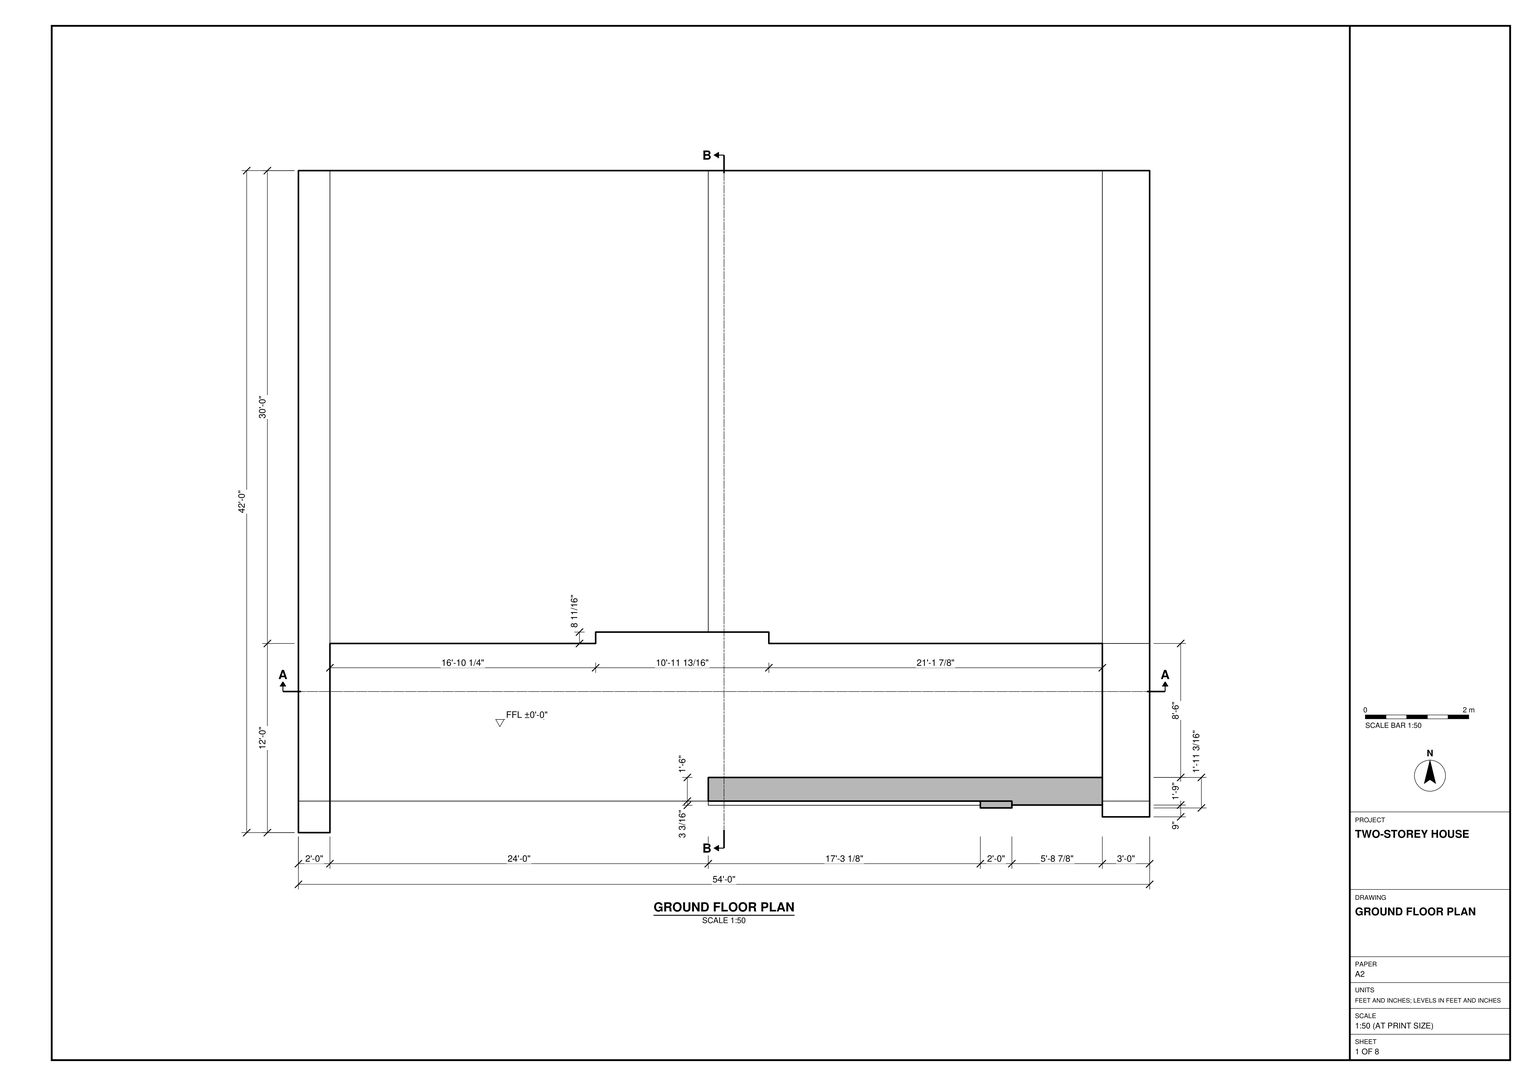
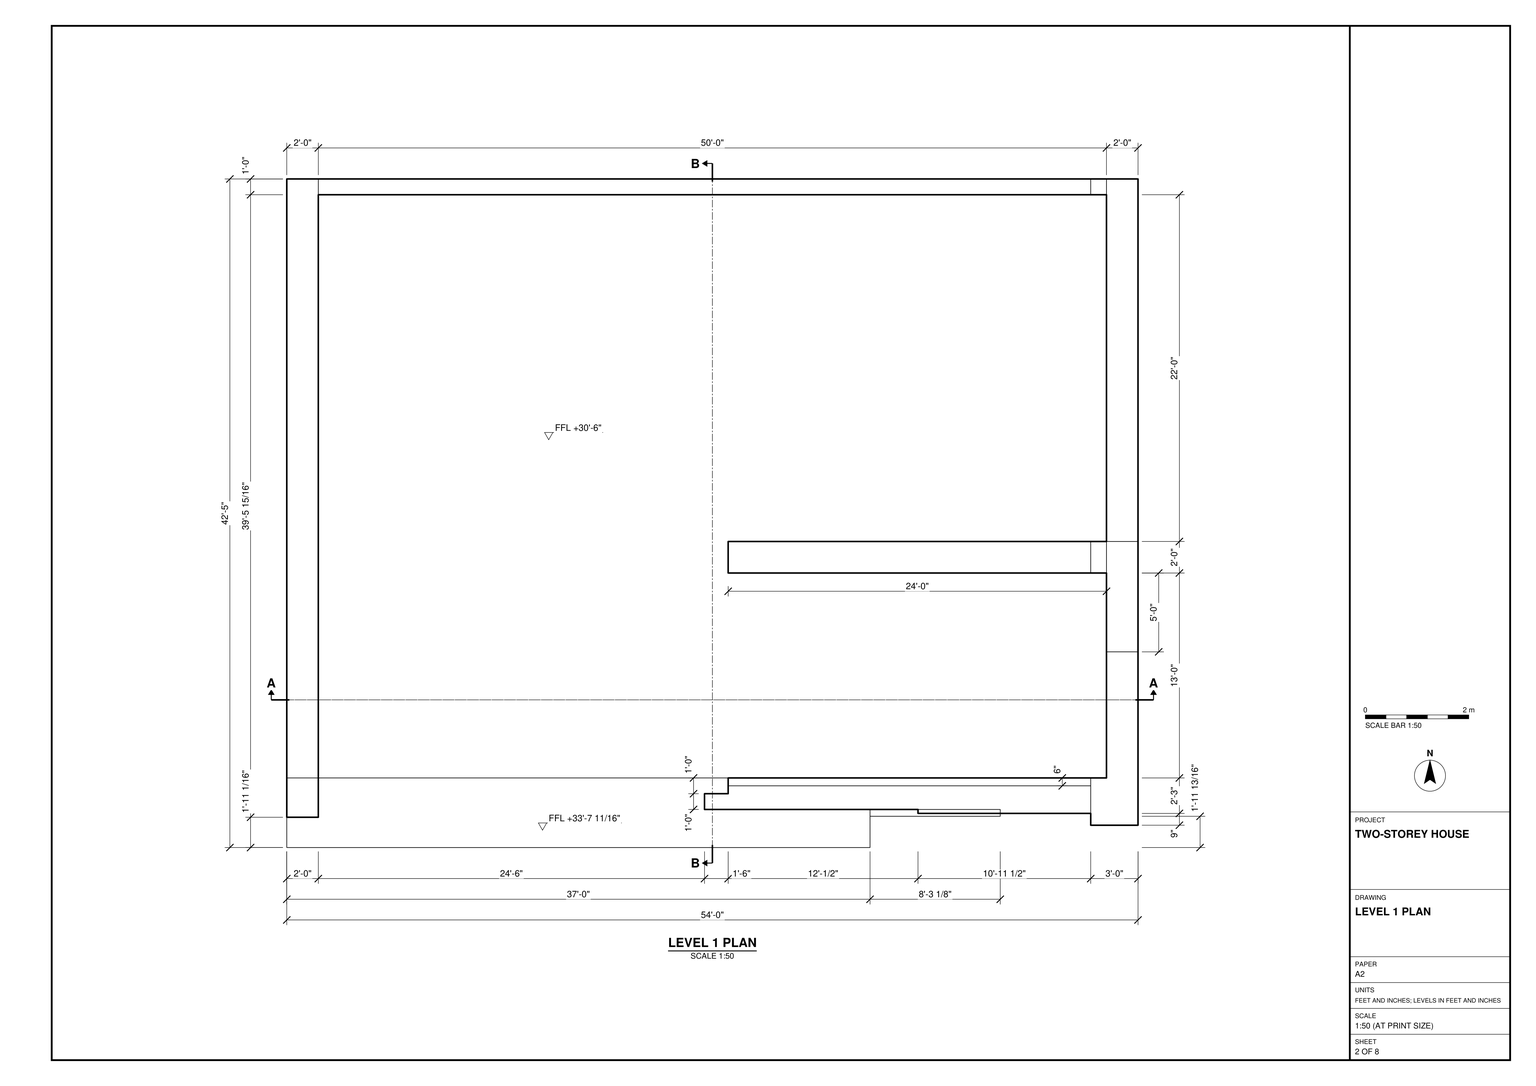
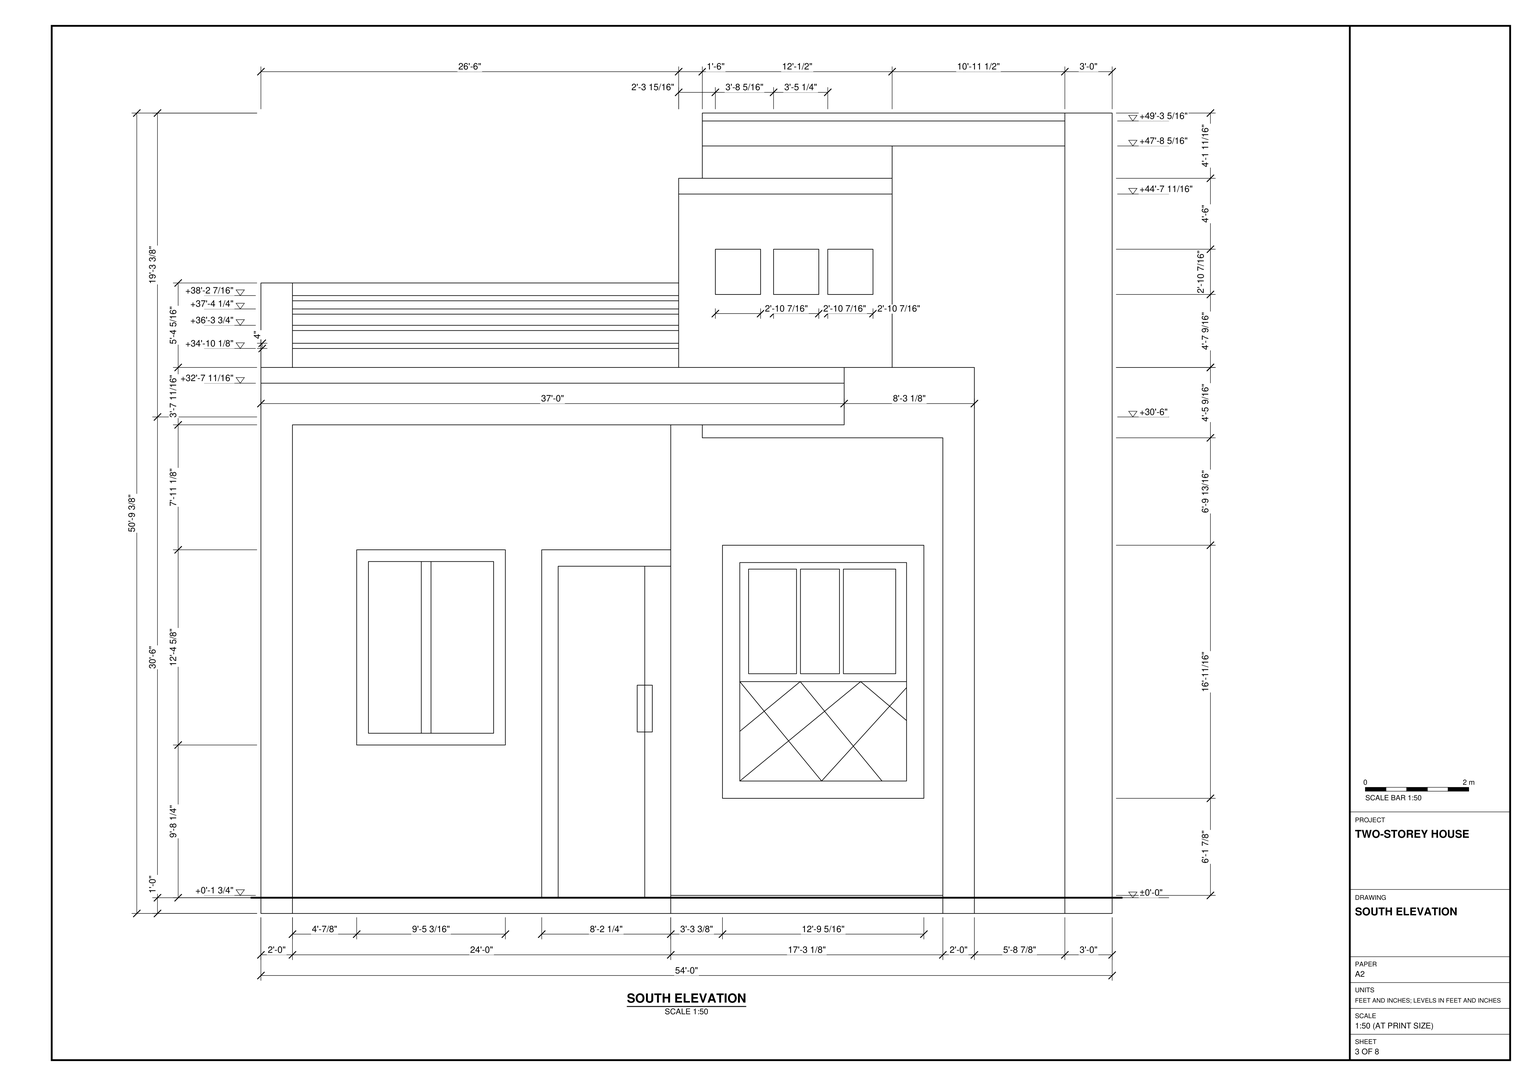
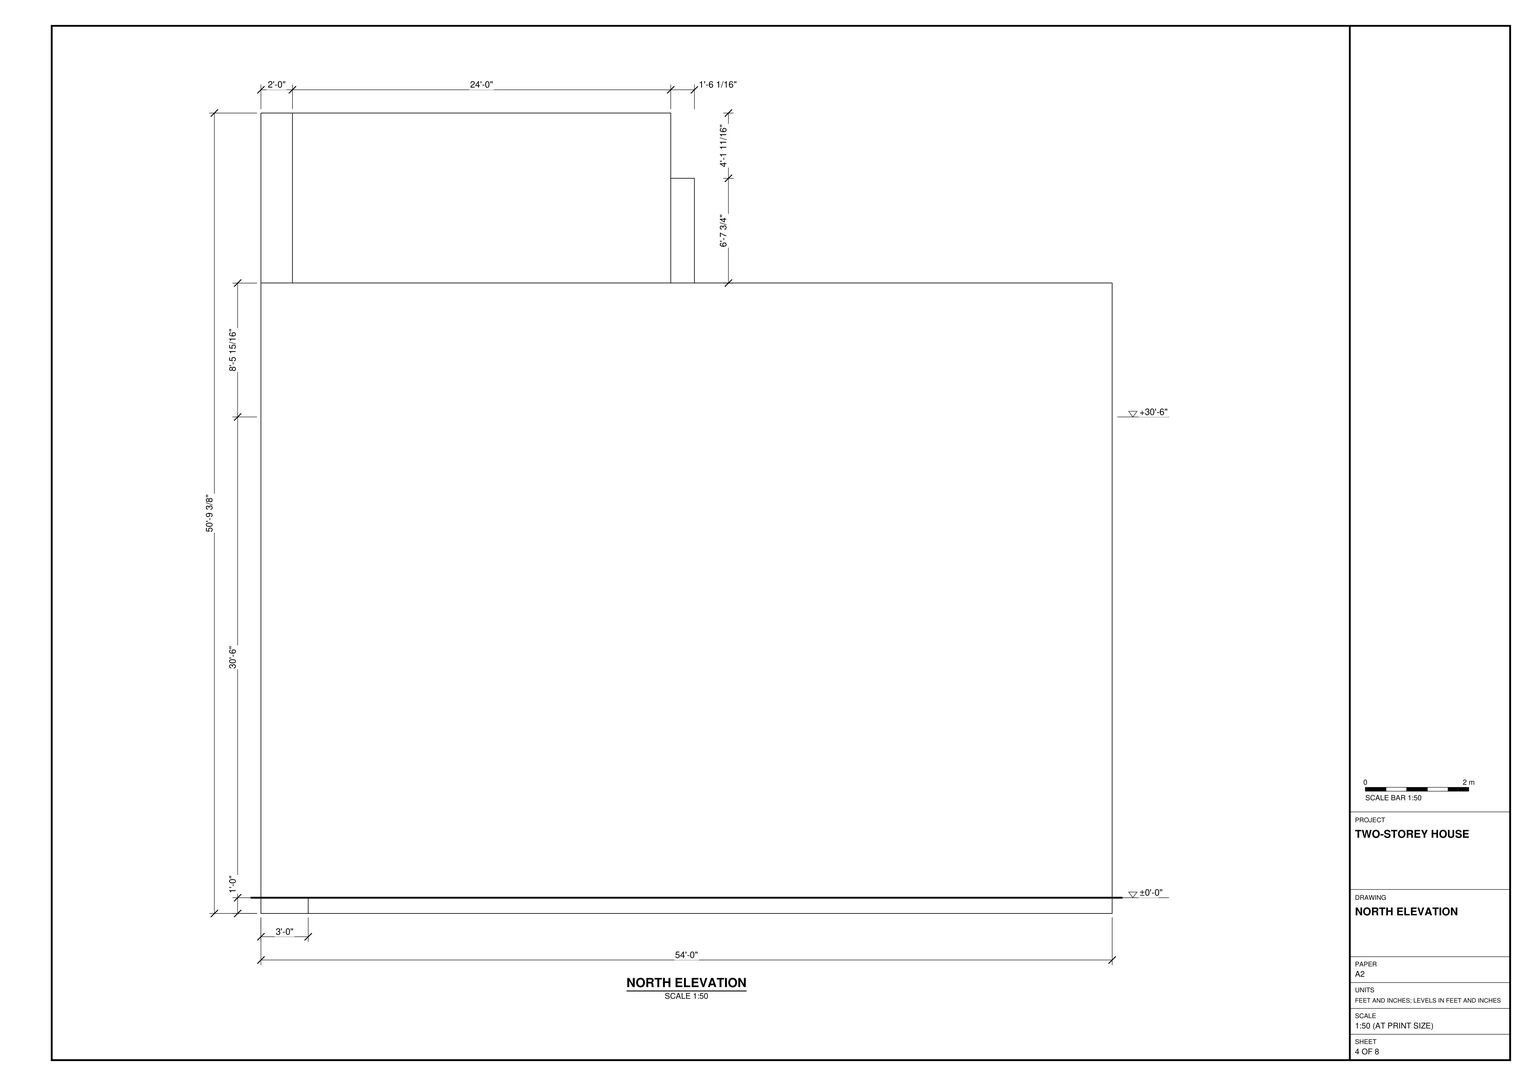
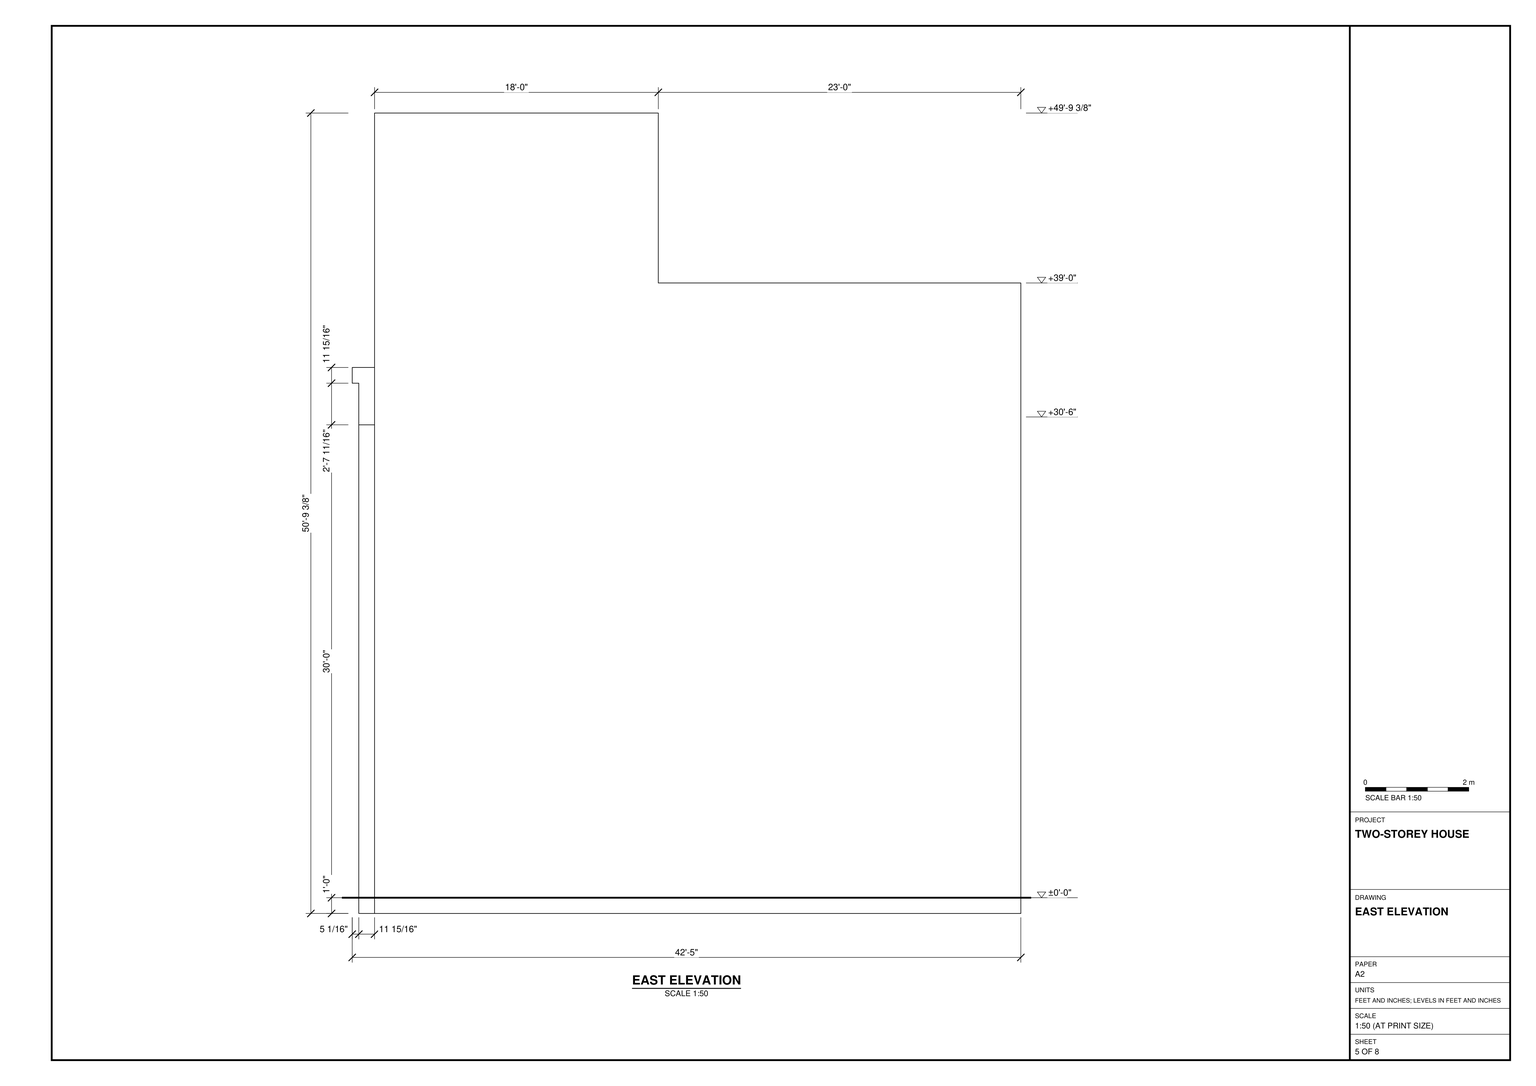
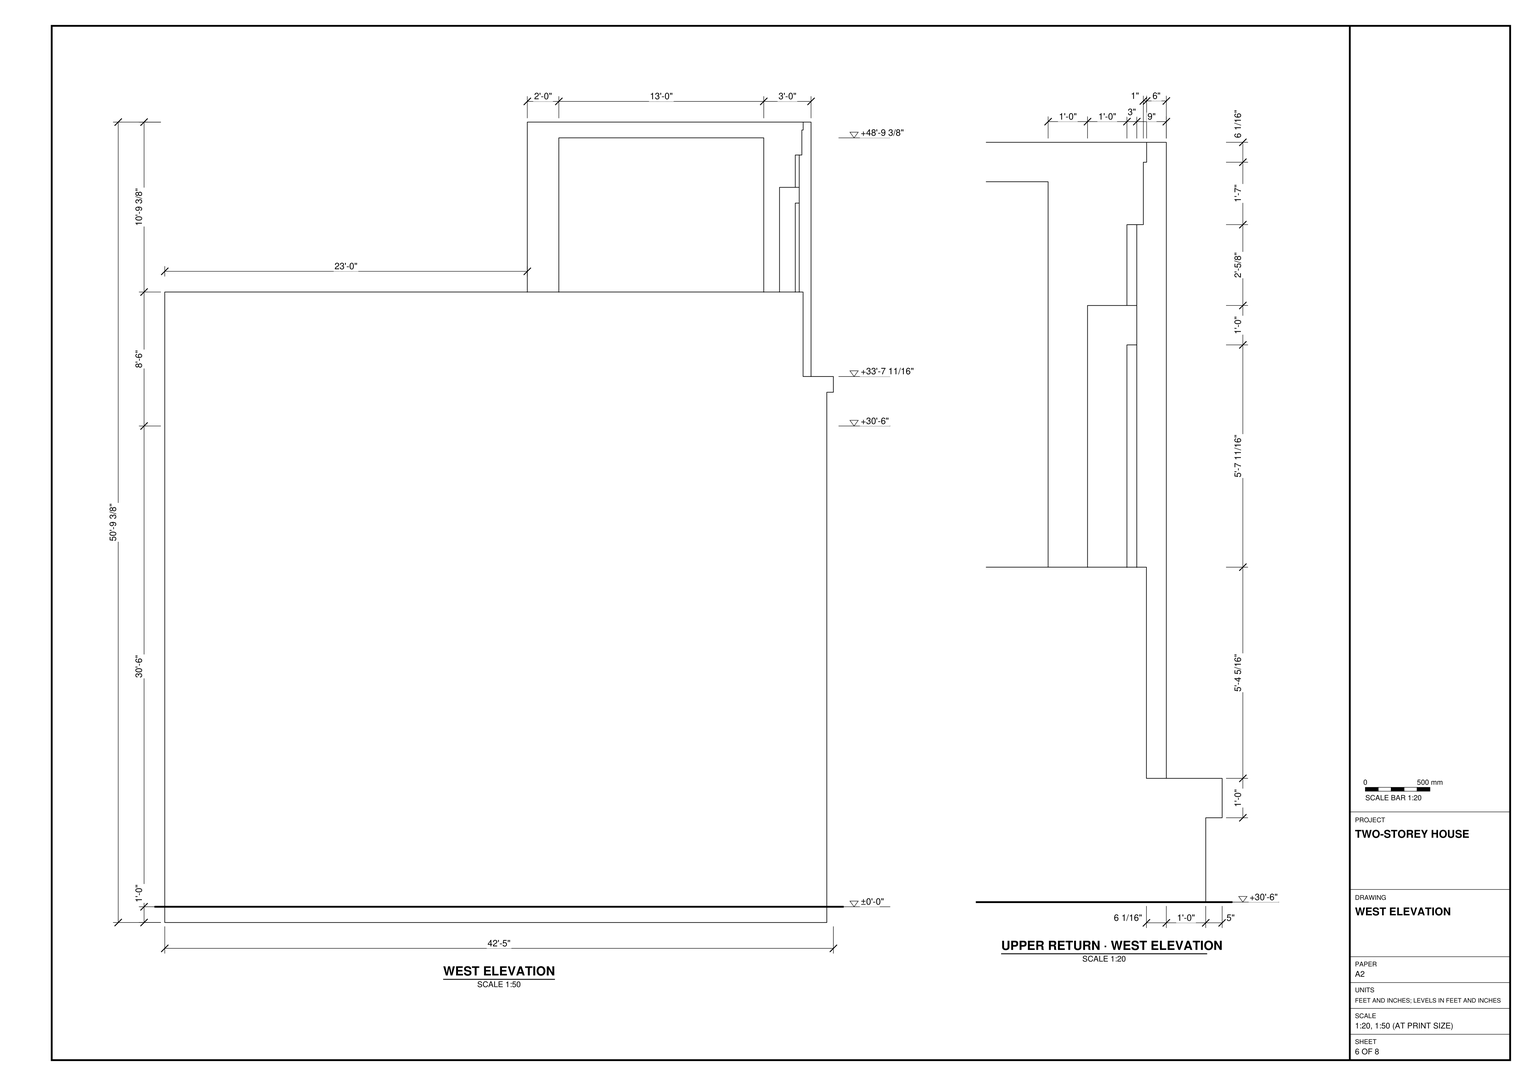
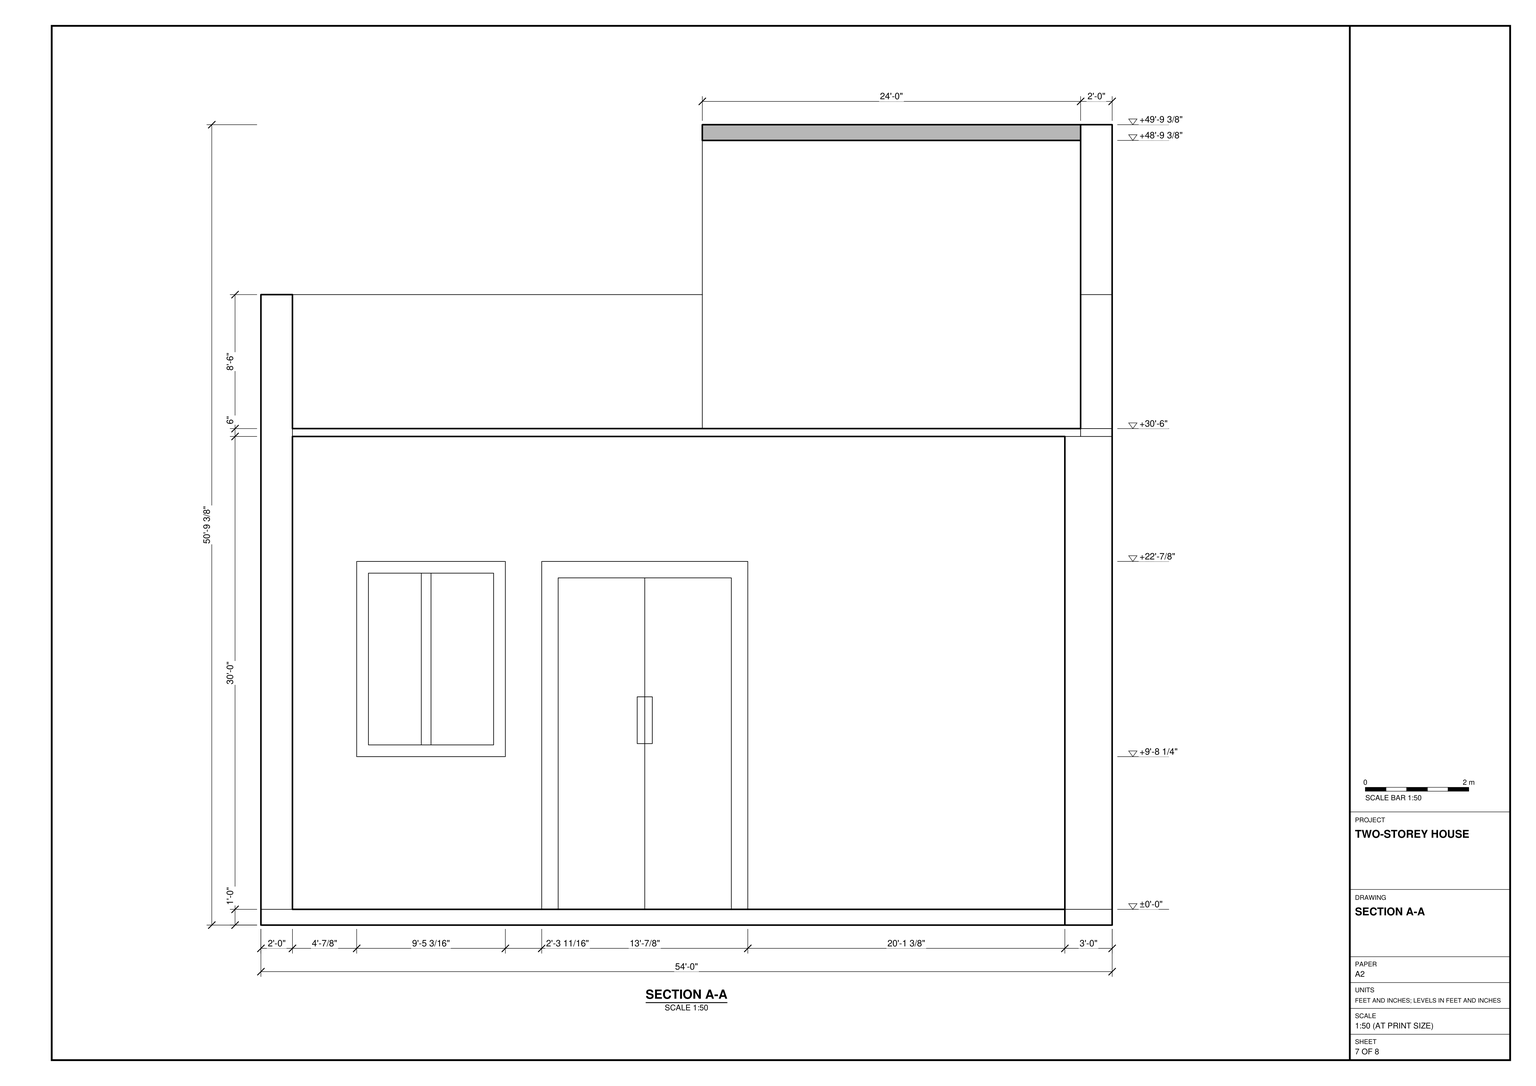
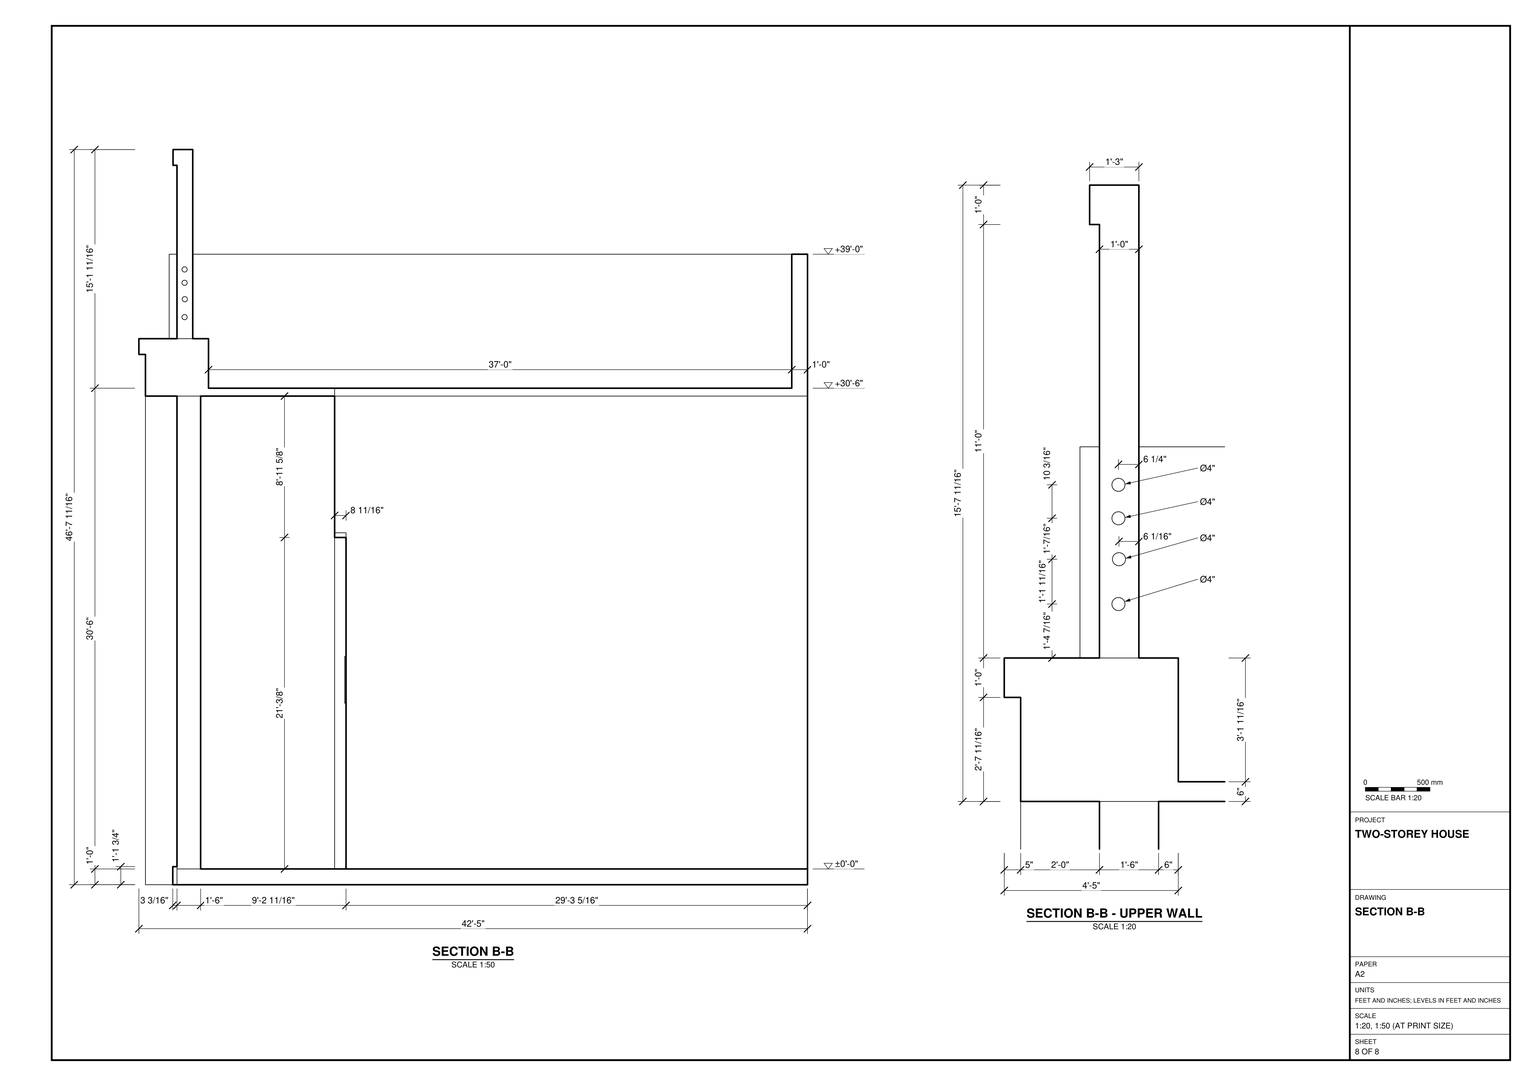
Model the house in SketchUp using task_files/diagram_01.pdf. Work in feet and inches. The overall dimensions are 54'-0" wide along X, 42'-5" deep along Y and 50'-9 3/8" high. Set the ground floor at ±0'-0" and the upper floor at +30'-6".

Use the plans to lay out the base, floor slabs and walls, following the wall thicknesses and changes in outline as drawn. On the south side, set the entrance wall back behind the side piers. Place the entrance door between the narrower divided window on the left and the larger framed window on the right. Model the upper panes and diagonal lower grille of the right-hand window. Carry the horizontal beam across the front and turn it down beside this window.

Follow the upper plan for the slab edges and the narrow return on the right. Match the stepped roof profile in the south elevation: the horizontal rails on the left meet a raised panel with three square openings, and the highest roof edge rises behind the panel to the right. Include stairs, built-in joinery and main furniture where shown. Keep shell elements such as walls, slabs and roof separate as groups or components, group each furniture or joinery piece separately, and use components for repeated parts. Decor and loose items may be any suitable library components. Save one SketchUp model as output_files/two_storey_house_with_a_stepped_south_facade.skp.

# SketchUp Ruby script. Lengths in inches.
U = 1.inch
M = Sketchup.active_model
def pt(a) = Geom::Point3d.new(a.map { |v| v * U })
def face(e, loops, mat)
  f = e.add_face(loops[0].map { |a| pt(a) })
  loops[1..].each { |l| e.add_face(l.map { |a| pt(a) }).erase! }
  f.material = f.back_material = mat if mat
  f
end
# faces: each face lists its corners as indices into pts; further lists are holes
def faces(e, pts, list, mat = nil) = list.each { |f| face(e, (f[0].is_a?(Array) ? f : [f]).map { |l| l.map { |i| pts[i] } }, mat) }
# xy, xz, yz: faces in a plane at the given z, y or x. An outline is a flat list of corners, or four numbers for a rectangle; further outlines are holes
def ring(l) = l.size == 4 ? [[l[0], l[1]], [l[2], l[1]], [l[2], l[3]], [l[0], l[3]]] : l.each_slice(2).to_a
def flat(e, list, mat, &to3) = list.each { |f| face(e, (f[0].is_a?(Array) ? f : [f]).map { |l| ring(l).map { |u, v| to3.(u, v) } }, mat) }
def xy(e, z, list, mat = nil) = flat(e, list, mat) { |x, y| [x, y, z] }
def xz(e, y, list, mat = nil) = flat(e, list, mat) { |x, z| [x, y, z] }
def yz(e, x, list, mat = nil) = flat(e, list, mat) { |y, z| [x, y, z] }
def lines(e, pts, list) = list.each { |a, b| e.add_line(pt(pts[a]), pt(pts[b])) }
# prism: a flat outline (further loops are holes) pulled along v
def prism(e, loops, v, mat = nil)
  f = face(e, loops, mat); d = Geom::Vector3d.new(v.map { |x| x * U })
  f.pushpull(f.normal.samedirection?(d) ? d.length : -d.length)
end
def box(e, o, s, mat = nil) = prism(e, [[o, [o[0] + s[0], o[1], o[2]], [o[0] + s[0], o[1] + s[1], o[2]], [o[0], o[1] + s[1], o[2]]]], [0, 0, s[2]], mat)
def at(x, y, z, deg = 0) = Geom::Transformation.translation(pt([x, y, z])) * Geom::Transformation.rotation(ORIGIN, Z_AXIS, deg.degrees)
def axes(o, x, y, z) = Geom::Transformation.new([*x, 0, *y, 0, *z, 0, *pt(o).to_a, 1])
def part(name) = M.definitions.add(name)
# library, detail: a bought-in or finely detailed component or shape, given as its bounding box
def library(name, o, s) = part(name).tap { |d| box(d.entities, o, s) }
def detail(e, o, s) = box(e.add_group.entities, o, s)
def put(e, d, t, mat = nil) = e.add_instance(d, t).tap { |i| i.material = mat if mat }
def group(e, t, mat = nil) = e.add_group.tap { |g| g.transformation = t; g.material = mat if mat }.entities
root = M.entities
M.materials.add("[0001_PaleVioletRed]").color = [219, 112, 147]
M.materials.add("[0009_Linen]").color = [186, 178, 171]
M.materials.add("[0023_FireBrick]").color = [71, 13, 13]
M.materials.add("[0035_Tan]").color = [114, 98, 76]
M.materials.add("[0042_Sienna]").color = [58, 30, 16]
M.materials.add("[0119_RosyBrown]").color = [124, 95, 95]
M.materials.add("[0134_DimGray]").color = [105, 105, 105]
M.materials.add("[0137_Black]").color = [0, 0, 0]
M.materials.add("[Asphalt New]").color = [67, 60, 62]
M.materials.add("[Granite Brown]").color = [126, 104, 91]
M.materials.add("[Translucent Glass Gray]").color = [128, 128, 128]
M.materials["[Translucent Glass Gray]"].alpha = 0.5
xy(root,0,[[0,5,24,29],[612,17,648,29],[519.125,23.8,543.125,29],[312,25.8,312,29,0,29,0,509,612,509,612,26,543.125,26,543.125,29,519.125,29,519.125,25.8],[612,29,648,509]])
xy(root,12,[[24,149,24,509,312,509,312,157.6875,226.28,157.6875,226.28,149],[358.11,149,358.11,157.6875,312,157.6875,312,509,612,509,612,149]])
xy(root,12,[[24,29,312,29,312,47,612,47,612,149,358.11,149,358.11,157.6875,226.28,157.6875,226.28,149,24,149]],"[Granite Brown]")
xy(root,13.76,[[312,25.8,519.125,29]])
xy(root,87.65,[[351.36,17,504.67,29]])
xy(root,100.83,[[364.54,17,491.5,29]])
xy(root,137.19,[[81.83,149,122.08,157.6875],[129.48,149,177.13,157.6875]])
xy(root,138.18,[[286.45,156.6875,292.2,157.6875],[292.2,156.6875,297.95,157.6875]])
xy(root,173.8,[[286.45,156.6875,292.2,157.6875],[292.2,156.6875,297.95,157.6875]])
xy(root,264.36,[[226.28,149,358.11,157.6875]])
xy(root,267.16,[[364.54,17,491.5,29]])
xy(root,267.93,[[81.83,149,122.08,157.6875],[129.48,149,177.13,157.6875]])
xy(root,280.34,[[351.36,17,504.67,29]])
xy(root,362.125,[[336,23.8,519.125,29]])
xy(root,372,[[24,5,24,149,612,149,612,47,312,47,312,29,336,29,336,23.8,444,23.8,444,5],[336,23.8,444,29]])
xy(root,378,[[24,53,624,53,624,209,336,209,336,233,624,233,624,497,24,497]])
xy(root,403.6875,[[0,0,444,5]])
xy(root,415.6875,[[444,23.8,543.125,23.8,543.125,26,480.51,26,480.51,29,444,29],[480.51,26,543.125,29]])
xy(root,415.6875,[[0,0,444,0,444,29,318,29,318,41,336,41,336,53,24,53,24,23.0625,0,23.0625]],"[Asphalt New]")
xy(root,430.13,[[24,34.5,318,35.02]])
xy(root,443.79,[[24,34.66,318,35.18]])
xy(root,460.22,[[24,34.54,318,35.06]])
xy(root,470.41,[[24,34.54,318,35.06]])
xy(root,471.25,[[345.95,29,380.38,31],[390.26,29,424.7,31],[431.51,29,465.95,31]],"[0137_Black]")
xy(root,480,[[0,23.0625,24,509],[624,233,648,233,648,509,24,509,24,497,624,497]])
xy(root,505.68,[[345.95,29,380.38,31],[390.26,29,424.7,31],[431.51,29,465.95,31]],"[0137_Black]")
xy(root,547.6875,[[318,26,480.51,29]])
xy(root,559.6875,[[318,26,480.51,26,480.51,29,336,29,336,41,318,41]])
xy(root,584.3125,[[336,24,336,29,480.51,29,480.51,26,612,26,612,24],[480.51,26,612,29]])
xy(root,597.375,[[336,53,624,209]])
xy(root,603.3125,[[336,23,612,24]])
xy(root,609.375,[[612,17,648,17,648,233,336,233,336,209,624,209,624,53,336,53,336,23,612,23],[336,53,624,209]])
xz(root,0,[[0,403.6875,444,415.6875]],"[Asphalt New]")
xz(root,5,[[0,0,24,0,24,372,444,372,444,403.6875,0,403.6875]],"[Asphalt New]")
xz(root,17,[[[351.36,87.65,504.67,280.34],[364.54,100.83,491.5,267.16]]],"[0035_Tan]")
xz(root,17,[[612,0,648,609.375]],"[Asphalt New]")
xz(root,23,[[336,603.3125,612,609.375]],"[Asphalt New]")
xz(root,23.0625,[[0,415.6875,24,480]])
xz(root,23.8,[[519.125,0,543.125,0,543.125,415.6875,444,415.6875,444,372,336,372,336,362.125,519.125,362.125]],"[0001_PaleVioletRed]")
xz(root,24,[[336,584.3125,612,603.3125]],"[Asphalt New]")
xz(root,25.8,[[312,0,519.125,13.76]],"[0134_DimGray]")
xz(root,26,[[318,547.6875,480.51,559.6875]])
xz(root,26,[[543.125,0,612,0,612,584.3125,480.51,584.3125,480.51,415.6875,543.125,415.6875]],"[0119_RosyBrown]")
xz(root,29,[[519.125,0,519.125,362.125,336,362.125,336,372,444,372,444,415.6875,543.125,415.6875,543.125,0],[[351.36,87.65,504.67,280.34],[364.54,100.83,491.5,267.16]],[371.23,182.52,407.73,262.16],[410.73,182.52,440.42,262.16],[443.42,182.52,483.25,262.16]])
xz(root,29,[[[312,13.76,519.125,13.76,519.125,362.125,336,362.125,336,372,312,372],[351.36,87.65,504.67,280.34]],[[318,415.6875,480.51,547.6875],[345.95,471.25,380.38,505.68],[390.26,471.25,424.7,505.68],[431.51,471.25,465.95,505.68]],[336,559.6875,480.51,584.3125]],"[0001_PaleVioletRed]")
xz(root,29,[[364.54,100.83,401.68,131.38,383.11,153.95,365.93,139.8125,364.54,138.67],[364.54,100.83,426.82,100.83,401.68,131.38],[426.82,100.83,450.96,127.39,429.1,153.95,401.68,131.38],[426.82,100.83,472.8125,100.83,450.96,127.39],[472.8125,100.83,491.5,100.83,491.5,146.88,478.6,157.81,450.96,127.39],
  [450.96,127.39,478.6,157.81,456.53,176.52,429.1,153.95],[401.68,131.38,429.1,153.95,410.54,176.52,383.11,153.95],[364.54,138.67,365.93,139.8125,383.11,153.95,364.54,176.52],[491.5,146.88,491.5,171.99,478.6,157.81],[383.11,153.95,410.54,176.52,364.54,176.52],
  [429.1,153.95,456.53,176.52,410.54,176.52],[478.6,157.81,491.5,171.99,491.5,176.52,456.53,176.52]],"[0009_Linen]")
xz(root,29,[[[364.54,176.52,491.5,267.16],[443.42,182.52,483.25,262.16],[371.23,182.52,407.73,262.16],[410.73,182.52,440.42,262.16]]],"[0137_Black]")
xz(root,29,[[24,0,312,12]],"[Granite Brown]")
xz(root,31,[[345.95,471.25,380.38,505.68],[390.26,471.25,424.7,505.68],[431.51,471.25,465.95,505.68]])
xz(root,36.76,[[24,431.83,318,432.36],[24,457.96,318,458.48],[24,468.15,318,468.67]])
xz(root,36.92,[[24,445.49,318,446.01]])
xz(root,41,[[318,415.6875,336,559.6875]])
xz(root,47,[[312,12,612,372]])
xz(root,53,[[24,378,24,415.6875,336,415.6875,336,597.375,624,597.375,624,378]])
xz(root,149,[[213.76,12,226.28,12,226.28,264.36,358.11,264.36,358.11,12,370.63,12,370.63,276.875,213.76,276.875]],"[0023_FireBrick]")
xz(root,149,[[[72.89,128.25,186.08,276.875],[81.83,137.19,177.13,267.93]],[122.08,137.19,129.48,267.93]],"[0137_Black]")
xz(root,149,[[[24,12,213.76,12,213.76,276.875,370.63,276.875,370.63,12,612,12,612,372,24,372],[72.89,128.25,186.08,276.875]]],"[Granite Brown]")
xz(root,156.6875,[[286.45,138.18,292.2,173.8],[292.2,138.18,297.95,173.8]])
xz(root,157.6875,[[226.28,12,292.2,12,292.2,138.18,286.45,138.18,286.45,173.8,292.2,173.8,292.2,264.36,226.28,264.36],[292.2,12,358.11,12,358.11,264.36,292.2,264.36,292.2,173.8,297.95,173.8,297.95,138.18,292.2,138.18]],"[0042_Sienna]")
xz(root,157.6875,[[81.83,137.19,122.08,267.93],[129.48,137.19,177.13,267.93]],"[Translucent Glass Gray]")
xz(root,209,[[336,378,624,597.375]])
xz(root,233,[[336,378,624,609.375],[624,480,648,609.375]])
xz(root,497,[[24,378,624,480]])
xz(root,509,[[0,0,612,12],[612,0,648,12],[0,12,648,480]])
yz(root,0,[[5,0,5,403.6875,0,403.6875,0,415.6875,23.0625,415.6875,23.0625,480,509,480,509,0]])
yz(root,24,[[5,0,29,0,29,12,149,12,149,372,5,372],[[53,378,497,378,497,480,23.0625,480,23.0625,415.6875,53,415.6875],[34.5,430.13,34,430.27,33.55,430.54,33.18,430.91,32.92,431.37,32.79,431.87,32.8,432.39,32.9375,432.9,33.2,433.35,33.58,433.71,34.03,433.97,34.54,434.1,35.06,434.09,35.5625,433.95,36.01,433.6875,36.375,433.32,36.63,432.86,36.76,432.36,36.76,431.83,36.62,431.33,36.35,430.88,35.98,430.52,35.53,430.26,35.02,430.13],[34.66,443.79,34.15,443.93,33.7,444.2,33.34,444.57,33.08,445.02,32.95,445.53,32.96,446.05,33.09,446.55,33.36,447,33.73,447.37,34.1875,447.625,34.69,447.76,35.22,447.75,35.72,447.61,36.17,447.35,36.53,446.97,36.79,446.52,36.92,446.01,36.92,445.49,36.78,444.99,36.51,444.54,36.14,444.17,35.68,443.92,35.18,443.79],[35.02,456.25,34.5,456.26,34,456.4,33.55,456.66,33.18,457.04,32.92,457.49,32.79,458,32.8,458.52,32.9375,459.02,33.2,459.47,33.58,459.84,34.03,460.09,34.54,460.22,35.06,460.22,35.5625,460.08,36.01,459.8125,36.375,459.44,36.63,458.99,36.76,458.48,36.76,457.96,36.62,457.46,36.35,457.01,35.98,456.64,35.53,456.38],[35.02,466.44,34.5,466.45,34,466.59,33.55,466.85,33.18,467.22,32.92,467.68,32.79,468.18,32.8,468.71,32.9375,469.21,33.2,469.66,33.58,470.02,34.03,470.28,34.54,470.41,35.06,470.41,35.5625,470.27,36.01,470,36.375,469.63,36.63,469.17,36.76,468.67,36.76,468.15,36.62,467.64,36.35,467.19,35.98,466.83,35.53,466.57]]])
yz(root,81.83,[[149,137.19,157.6875,267.93]])
yz(root,122.08,[[149,137.19,157.6875,267.93]])
yz(root,129.48,[[149,137.19,157.6875,267.93]])
yz(root,177.13,[[149,137.19,157.6875,267.93]])
yz(root,226.28,[[149,12,157.6875,264.36]])
yz(root,286.45,[[156.6875,138.18,157.6875,173.8]])
yz(root,297.95,[[156.6875,138.18,157.6875,173.8]])
yz(root,312,[[25.8,0,29,13.76],[29,12,47,372]])
yz(root,318,[[[29,415.6875,29,547.6875,26,547.6875,26,559.6875,41,559.6875,41,415.6875],[34.5,430.13,35.02,430.13,35.53,430.26,35.98,430.52,36.35,430.88,36.62,431.33,36.76,431.83,36.76,432.36,36.63,432.86,36.375,433.32,36.01,433.6875,35.5625,433.95,35.06,434.09,34.54,434.1,34.03,433.97,33.58,433.71,33.2,433.35,32.9375,432.9,32.8,432.39,32.79,431.87,32.92,431.37,33.18,430.91,33.55,430.54,34,430.27],[35.02,466.44,35.53,466.57,35.98,466.83,36.35,467.19,36.62,467.64,36.76,468.15,36.76,468.67,36.63,469.17,36.375,469.63,36.01,470,35.5625,470.27,35.06,470.41,34.54,470.41,34.03,470.28,33.58,470.02,33.2,469.66,32.9375,469.21,32.8,468.71,32.79,468.18,32.92,467.68,33.18,467.22,33.55,466.85,34,466.59,34.5,466.45],[35.02,456.25,35.53,456.38,35.98,456.64,36.35,457.01,36.62,457.46,36.76,457.96,36.76,458.48,36.63,458.99,36.375,459.44,36.01,459.8125,35.5625,460.08,35.06,460.22,34.54,460.22,34.03,460.09,33.58,459.84,33.2,459.47,32.9375,459.02,32.8,458.52,32.79,458,32.92,457.49,33.18,457.04,33.55,456.66,34,456.4,34.5,456.26],[34.66,443.79,35.18,443.79,35.68,443.92,36.14,444.17,36.51,444.54,36.78,444.99,36.92,445.49,36.92,446.01,36.79,446.52,36.53,446.97,36.17,447.35,35.72,447.61,35.22,447.75,34.69,447.76,34.1875,447.625,33.73,447.37,33.36,447,33.09,446.55,32.96,446.05,32.95,445.53,33.08,445.02,33.34,444.57,33.7,444.2,34.15,443.93]],[34.5,430.13,35.02,430.13,35.53,430.26,35.98,430.52,36.35,430.88,36.62,431.33,36.76,431.83,36.76,432.36,36.63,432.86,36.375,433.32,36.01,433.6875,35.5625,433.95,35.06,434.09,34.54,434.1,34.03,433.97,33.58,433.71,33.2,433.35,32.9375,432.9,32.8,432.39,32.79,431.87,32.92,431.37,33.18,430.91,33.55,430.54,34,430.27],[34.66,443.79,35.18,443.79,35.68,443.92,36.14,444.17,36.51,444.54,36.78,444.99,36.92,445.49,36.92,446.01,36.79,446.52,36.53,446.97,36.17,447.35,35.72,447.61,35.22,447.75,34.69,447.76,34.1875,447.625,33.73,447.37,33.36,447,33.09,446.55,32.96,446.05,32.95,445.53,33.08,445.02,33.34,444.57,33.7,444.2,34.15,443.93],[35.02,456.25,35.53,456.38,35.98,456.64,36.35,457.01,36.62,457.46,36.76,457.96,36.76,458.48,36.63,458.99,36.375,459.44,36.01,459.8125,35.5625,460.08,35.06,460.22,34.54,460.22,34.03,460.09,33.58,459.84,33.2,459.47,32.9375,459.02,32.8,458.52,32.79,458,32.92,457.49,33.18,457.04,33.55,456.66,34,456.4,34.5,456.26],[35.02,466.44,35.53,466.57,35.98,466.83,36.35,467.19,36.62,467.64,36.76,468.15,36.76,468.67,36.63,469.17,36.375,469.63,36.01,470,35.5625,470.27,35.06,470.41,34.54,470.41,34.03,470.28,33.58,470.02,33.2,469.66,32.9375,469.21,32.8,468.71,32.79,468.18,32.92,467.68,33.18,467.22,33.55,466.85,34,466.59,34.5,466.45]])
yz(root,336,[[23.8,362.125,29,372],[209,378,209,597.375,53,597.375,53,415.6875,41,415.6875,41,559.6875,29,559.6875,29,584.3125,24,584.3125,24,603.3125,23,603.3125,23,609.375,233,609.375,233,378]])
yz(root,345.95,[[29,471.25,31,505.68]],"[0137_Black]")
yz(root,351.36,[[17,87.65,29,280.34]])
yz(root,358.11,[[149,12,157.6875,264.36]])
yz(root,364.54,[[17,100.83,29,267.16]])
yz(root,380.38,[[29,471.25,31,505.68]],"[0137_Black]")
yz(root,390.26,[[29,471.25,31,505.68]],"[0137_Black]")
yz(root,424.7,[[29,471.25,31,505.68]],"[0137_Black]")
yz(root,431.51,[[29,471.25,31,505.68]],"[0137_Black]")
yz(root,444,[[5,372,23.8,372,23.8,415.6875,0,415.6875,0,403.6875,5,403.6875],[23.8,372,29,415.6875]])
yz(root,465.95,[[29,471.25,31,505.68]],"[0137_Black]")
yz(root,480.51,[[26,415.6875,29,547.6875],[26,559.6875,29,584.3125]],"[0119_RosyBrown]")
yz(root,491.5,[[17,100.83,29,267.16]])
yz(root,504.67,[[17,87.65,29,280.34]])
yz(root,519.125,[[23.8,0,25.8,13.76],[25.8,0,29,13.76],[23.8,13.76,29,362.125]])
yz(root,543.125,[[23.8,0,26,12],[26,0,29,12],[23.8,12,26,415.6875],[26,12,29,415.6875]])
yz(root,612,[[26,0,509,12],[26,12,47,372],[47,12,149,372],[24,584.3125,29,603.3125]])
yz(root,612,[[17,0,17,609.375,23,609.375,23,603.3125,24,603.3125,24,584.3125,26,584.3125,26,0]],"[Asphalt New]")
yz(root,624,[[53,378,209,597.375],[233,378,497,480],[53,597.375,209,609.375]])
yz(root,648,[[17,0,509,0,509,480,233,480,233,609.375,17,609.375]])
p = [[318,34.5,430.13],[318,34,430.27],[24,34,430.27],[24,34.5,430.13],[318,35.53,430.26],[318,35.02,430.13],
  [24,35.02,430.13],[24,35.53,430.26],[318,33.55,430.54],[24,33.55,430.54],[318,35.98,430.52],[24,35.98,430.52],
  [318,33.18,430.91],[24,33.18,430.91],[318,36.35,430.88],[24,36.35,430.88],[318,32.92,431.37],[24,32.92,431.37],
  [318,36.62,431.33],[24,36.62,431.33],[318,36.76,431.83],[24,36.76,431.83],[318,32.79,431.87],[24,32.79,431.87],
  [318,32.8,432.39],[24,32.8,432.39],[318,32.9375,432.9],[24,32.9375,432.9],[318,36.63,432.86],[318,36.76,432.36],
  [24,36.76,432.36],[24,36.63,432.86],[318,33.2,433.35],[24,33.2,433.35],[318,36.375,433.32],[24,36.375,433.32],
  [318,33.58,433.71],[24,33.58,433.71],[318,36.01,433.6875],[24,36.01,433.6875],[318,34.03,433.97],[24,34.03,433.97],
  [318,35.5625,433.95],[24,35.5625,433.95],[318,34.54,434.1],[24,34.54,434.1],[318,35.06,434.09],[24,35.06,434.09],
  [318,34.66,443.79],[318,34.15,443.93],[24,34.15,443.93],[24,34.66,443.79],[318,35.68,443.92],[318,35.18,443.79],
  [24,35.18,443.79],[24,35.68,443.92],[318,33.7,444.2],[24,33.7,444.2],[318,36.14,444.17],[24,36.14,444.17],
  [318,33.34,444.57],[24,33.34,444.57],[318,36.51,444.54],[24,36.51,444.54],[318,36.78,444.99],[24,36.78,444.99],
  [318,33.08,445.02],[24,33.08,445.02],[318,32.95,445.53],[24,32.95,445.53],[318,36.92,445.49],[24,36.92,445.49],
  [318,32.96,446.05],[24,32.96,446.05],[318,36.79,446.52],[318,36.92,446.01],[24,36.92,446.01],[24,36.79,446.52],
  [318,33.09,446.55],[24,33.09,446.55],[318,36.53,446.97],[24,36.53,446.97],[318,33.36,447],[24,33.36,447],
  [318,33.73,447.37],[24,33.73,447.37],[318,36.17,447.35],[24,36.17,447.35],[318,35.72,447.61],[24,35.72,447.61],
  [318,34.1875,447.625],[24,34.1875,447.625],[318,34.69,447.76],[24,34.69,447.76],[318,35.22,447.75],[24,35.22,447.75],
  [318,34.5,456.26],[318,34,456.4],[24,34,456.4],[24,34.5,456.26],[318,35.02,456.25],[24,35.02,456.25],
  [318,35.53,456.38],[24,35.53,456.38],[318,33.55,456.66],[24,33.55,456.66],[318,35.98,456.64],[24,35.98,456.64],
  [318,36.35,457.01],[24,36.35,457.01],[318,33.18,457.04],[24,33.18,457.04],[318,32.92,457.49],[24,32.92,457.49],
  [318,36.62,457.46],[24,36.62,457.46],[318,32.79,458],[24,32.79,458],[318,36.76,457.96],[24,36.76,457.96],
  [318,32.8,458.52],[24,32.8,458.52],[318,32.9375,459.02],[24,32.9375,459.02],[318,36.63,458.99],[318,36.76,458.48],
  [24,36.76,458.48],[24,36.63,458.99],[318,33.2,459.47],[24,33.2,459.47],[318,36.375,459.44],[24,36.375,459.44],
  [318,36.01,459.8125],[24,36.01,459.8125],[318,33.58,459.84],[24,33.58,459.84],[318,34.03,460.09],[24,34.03,460.09],
  [318,35.5625,460.08],[24,35.5625,460.08],[318,34.54,460.22],[24,34.54,460.22],[318,35.06,460.22],[24,35.06,460.22],
  [318,34.5,466.45],[318,34,466.59],[24,34,466.59],[24,34.5,466.45],[318,35.02,466.44],[24,35.02,466.44],
  [318,35.53,466.57],[24,35.53,466.57],[318,33.55,466.85],[24,33.55,466.85],[318,35.98,466.83],[24,35.98,466.83],
  [318,36.35,467.19],[24,36.35,467.19],[318,33.18,467.22],[24,33.18,467.22],[318,32.92,467.68],[24,32.92,467.68],
  [318,36.62,467.64],[24,36.62,467.64],[318,36.76,468.15],[24,36.76,468.15],[318,32.79,468.18],[24,32.79,468.18],
  [318,32.8,468.71],[24,32.8,468.71],[318,32.9375,469.21],[24,32.9375,469.21],[318,36.63,469.17],[318,36.76,468.67],
  [24,36.76,468.67],[24,36.63,469.17],[318,33.2,469.66],[24,33.2,469.66],[318,36.375,469.63],[24,36.375,469.63],
  [318,36.01,470],[24,36.01,470],[318,33.58,470.02],[24,33.58,470.02],[318,34.03,470.28],[24,34.03,470.28],
  [318,35.5625,470.27],[24,35.5625,470.27],[318,34.54,470.41],[24,34.54,470.41],[318,35.06,470.41],[24,35.06,470.41],
  [24,509,372],[24,149,372],[0,29,12],[24,29,12],[24,149,378],[612,149,12],
  [648,149,12],[612,149,372],[612,509,372],[624,149,372],[624,509,372],[624,149,378],
  [648,149,372],[612,29,603.3125],[612,29,609.375],[24,53,415.6875],[0,53,415.6875],[336,29,603.3125],
  [24,53,378],[0,53,378],[624,233,378],[648,233,378],[318,34.78,432.11],[24,34.78,432.11],
  [318,34.94,445.77],[24,34.94,445.77],[318,34.78,458.24],[24,34.78,458.24],[318,34.78,468.43],[24,34.78,468.43]]
faces(root,p,[[0,1,2,3],[4,5,6,7],[1,8,9,2],[10,4,7,11],[8,12,13,9],[14,10,11,15],[12,16,17,13],[18,14,15,19],
  [20,18,19,21],[16,22,23,17],[22,24,25,23],[24,26,27,25],[28,29,30,31],[26,32,33,27],[34,28,31,35],[32,36,37,33],
  [38,34,35,39],[36,40,41,37],[42,38,39,43],[40,44,45,41],[46,42,43,47],[44,46,47,45],[48,49,50,51],[52,53,54,55],
  [49,56,57,50],[58,52,55,59],[56,60,61,57],[62,58,59,63],[64,62,63,65],[60,66,67,61],[66,68,69,67],[70,64,65,71],
  [68,72,73,69],[74,75,76,77],[72,78,79,73],[80,74,77,81],[78,82,83,79],[82,84,85,83],[86,80,81,87],[88,86,87,89],
  [84,90,91,85],[90,92,93,91],[94,88,89,95],[92,94,95,93],[96,97,98,99],[100,96,99,101],[102,100,101,103],[97,104,105,98],
  [106,102,103,107],[108,106,107,109],[104,110,111,105],[110,112,113,111],[114,108,109,115],[112,116,117,113],[118,114,115,119],[116,120,121,117],
  [120,122,123,121],[124,125,126,127],[122,128,129,123],[130,124,127,131],[132,130,131,133],[128,134,135,129],[134,136,137,135],[138,132,133,139],
  [136,140,141,137],[142,138,139,143],[144,145,146,147],[148,144,147,149],[150,148,149,151],[145,152,153,146],[154,150,151,155],[156,154,155,157],
  [152,158,159,153],[158,160,161,159],[162,156,157,163],[164,162,163,165],[160,166,167,161],[166,168,169,167],[168,170,171,169],[172,173,174,175],
  [170,176,177,171],[178,172,175,179],[180,178,179,181],[176,182,183,177],[182,184,185,183],[186,180,181,187],[184,188,189,185],[190,186,187,191]])
lines(root,p,[[192,193],[194,195],[193,196],[197,198],[199,200],[201,202],[201,203],[199,201],[201,204],[205,206],[207,208],[205,209],
  [210,211],[212,213],[214,215],[216,217],[218,219],[220,221]])
